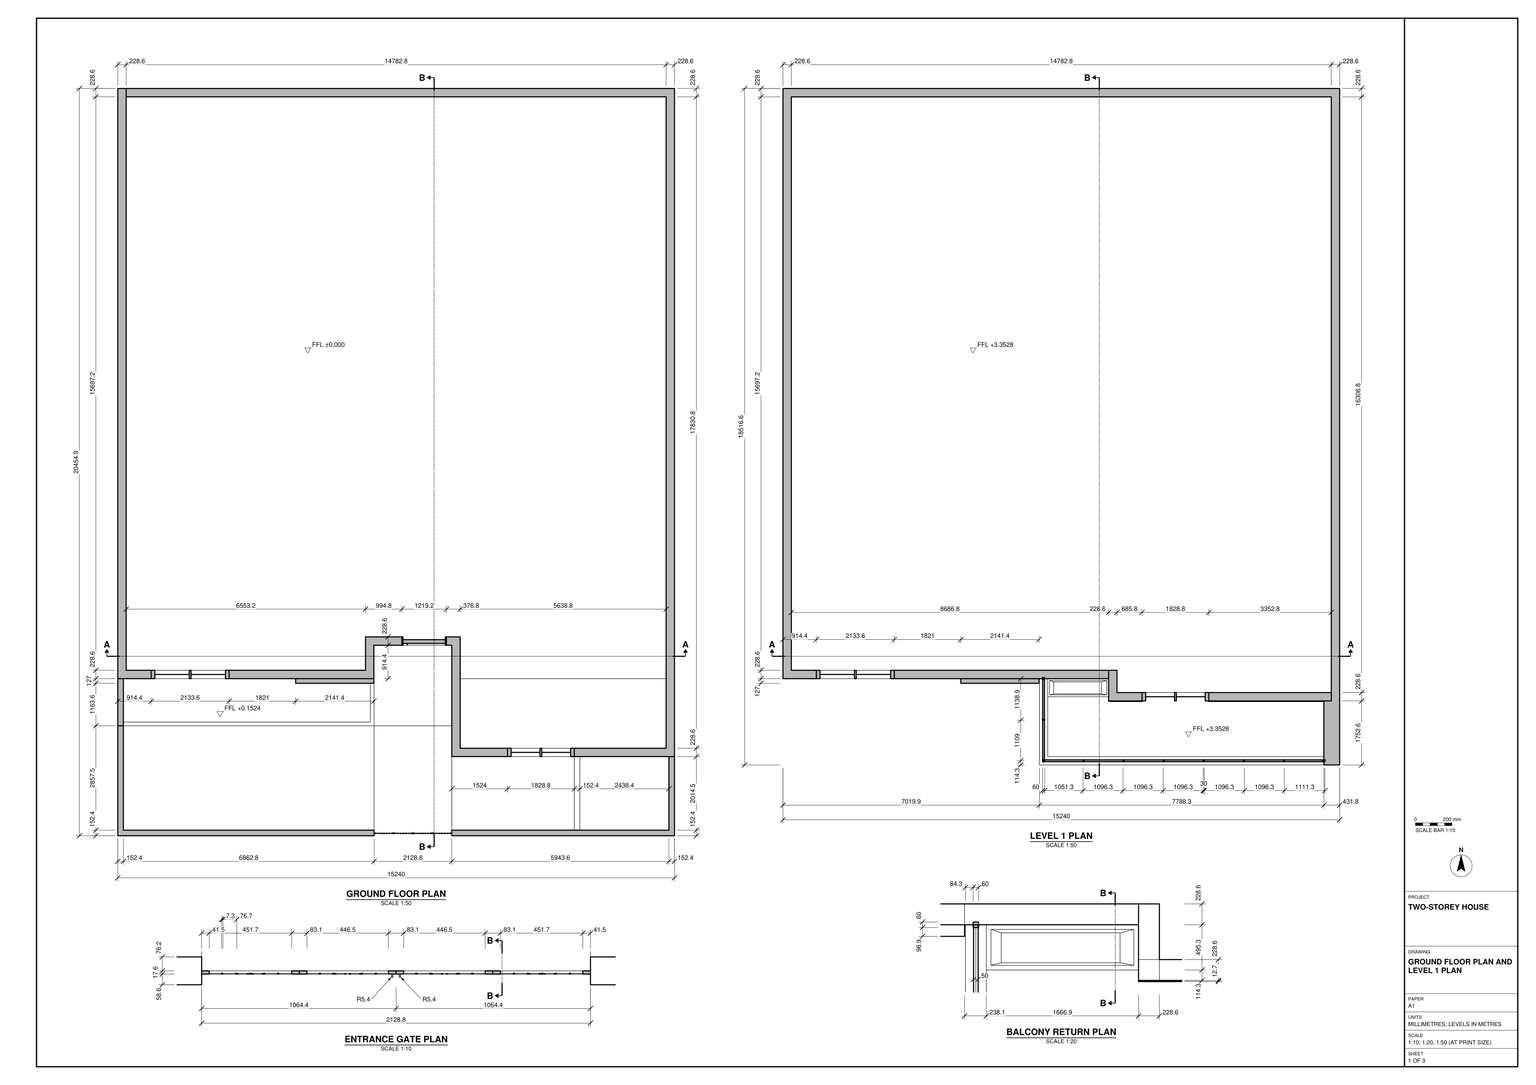
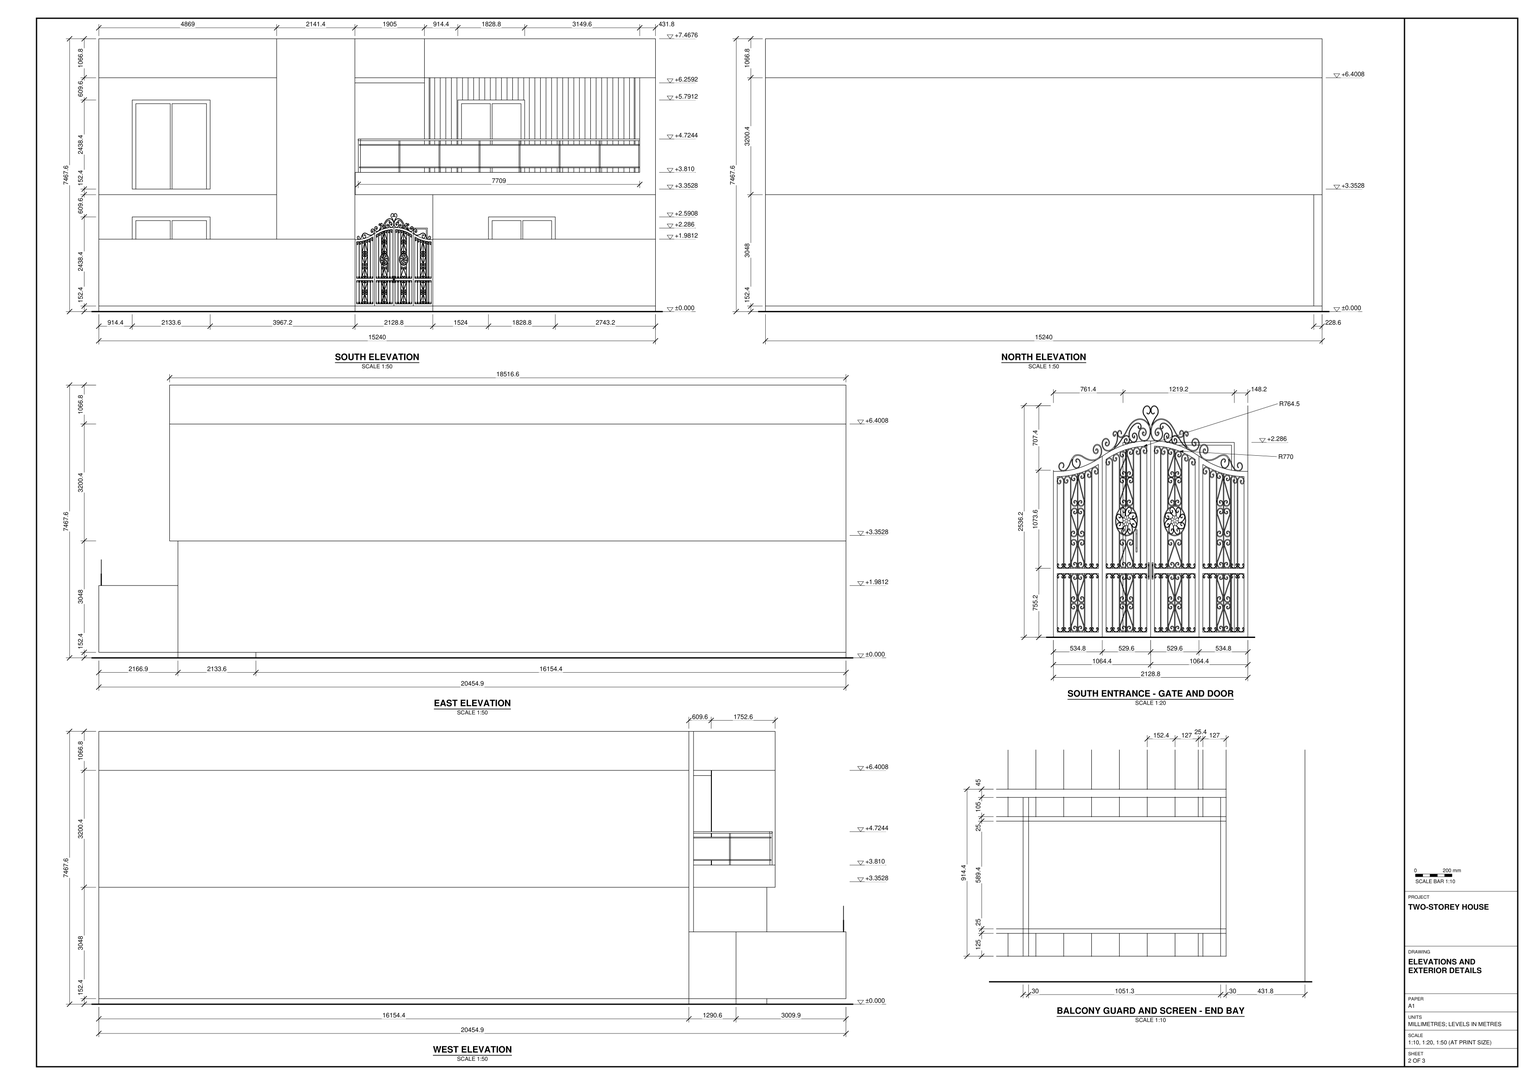
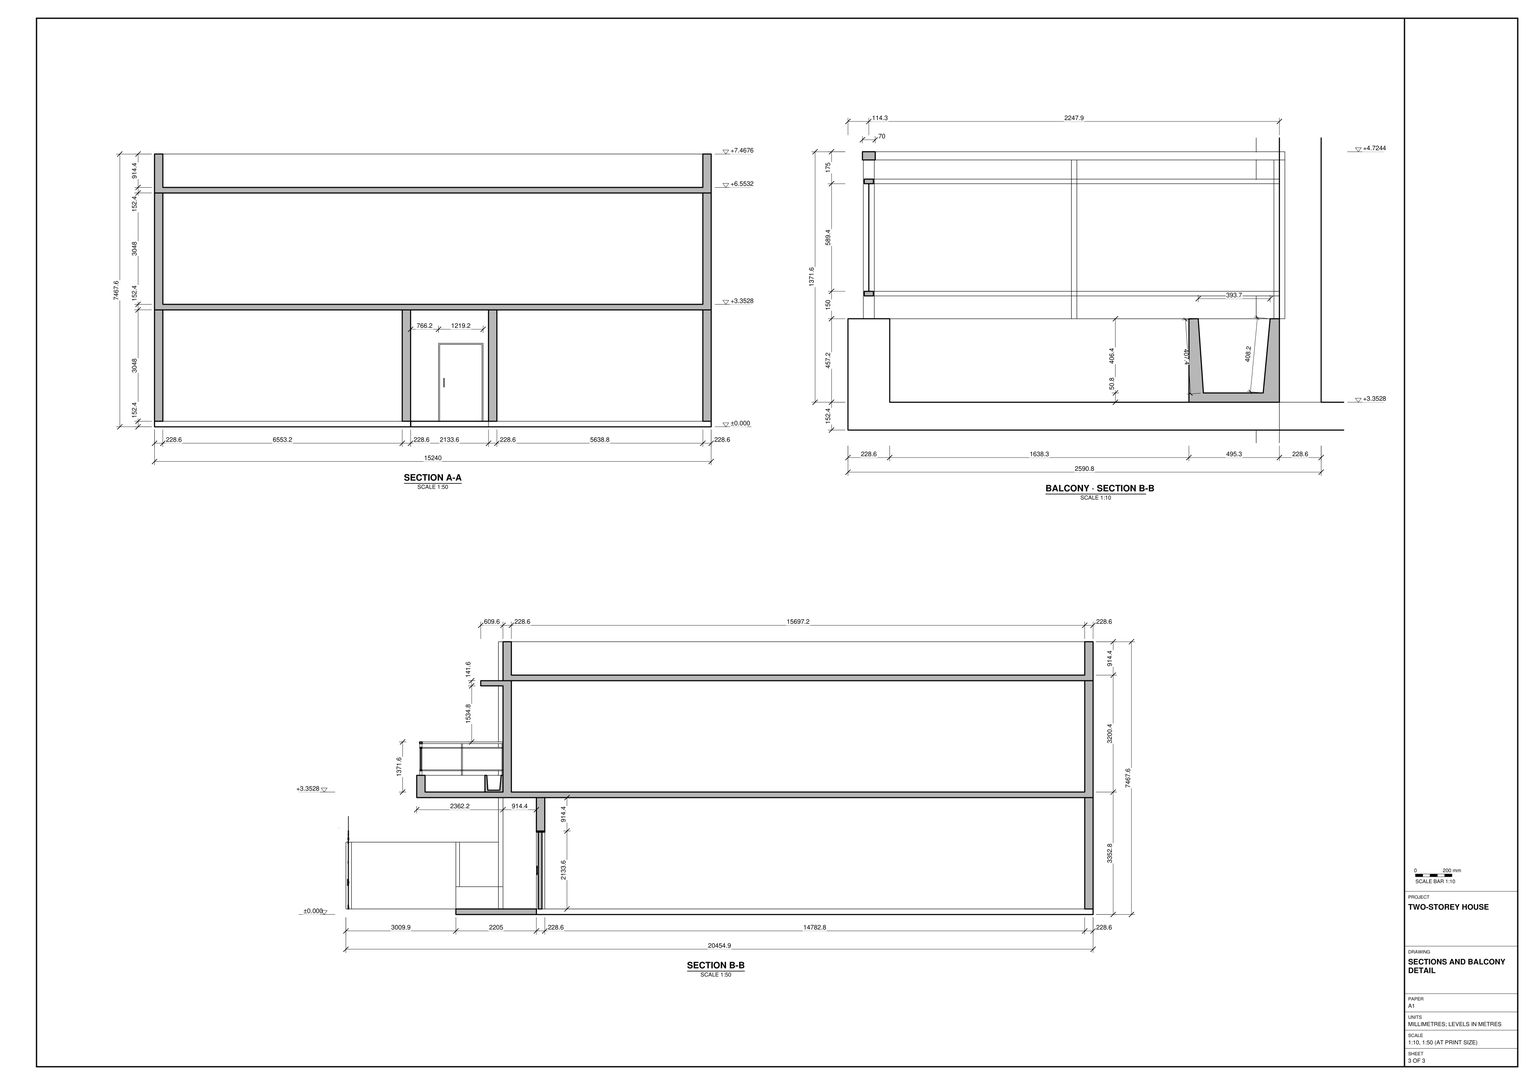
Build the house in SketchUp from task_files/diagram_01.pdf. Work in millimetres. Including the front enclosure, the model is 15240 mm wide, 20454.9 mm deep and 7467.6 mm high. Use 0 mm as the ground-floor datum and +3352.8 mm as the upper-floor level.

Follow the plans for the stepped south frontage: the entrance door sits in a recess, the eastern bay projects forward, and a double-leaf gate closes the gap between the low front walls. Model the exterior walls at their drawn thicknesses, the floor slabs, and the flat roof with its raised parapet. Keep the main floor areas open as drawn. Use the south elevation to place the framed openings on both storeys and to shape the curved crest and scrollwork of the gate.

Build the upper balcony on the eastern part of the south frontage. Use the enlarged plan and section to form the low balcony edge, the guard and its side return, and the recessed trough at the return. Include the vertical screen behind the guard. Keep shell elements and each furniture or joinery piece separate as groups or components, and use components for repeated parts. Any decor or loose items may be suitable library components. Save one SketchUp model as output_files/two_storey_house_with_a_gated_entrance_and_balcony.skp.

# SketchUp Ruby script. Lengths in millimetres.
U = 1.mm
M = Sketchup.active_model
def pt(a) = Geom::Point3d.new(a.map { |v| v * U })
def face(e, loops, mat)
  f = e.add_face(loops[0].map { |a| pt(a) })
  loops[1..].each { |l| e.add_face(l.map { |a| pt(a) }).erase! }
  f.material = f.back_material = mat if mat
  f
end
# faces: each face lists its corners as indices into pts; further lists are holes
def faces(e, pts, list, mat = nil) = list.each { |f| face(e, (f[0].is_a?(Array) ? f : [f]).map { |l| l.map { |i| pts[i] } }, mat) }
# xy, xz, yz: faces in a plane at the given z, y or x. An outline is a flat list of corners, or four numbers for a rectangle; further outlines are holes
def ring(l) = l.size == 4 ? [[l[0], l[1]], [l[2], l[1]], [l[2], l[3]], [l[0], l[3]]] : l.each_slice(2).to_a
def flat(e, list, mat, &to3) = list.each { |f| face(e, (f[0].is_a?(Array) ? f : [f]).map { |l| ring(l).map { |u, v| to3.(u, v) } }, mat) }
def xy(e, z, list, mat = nil) = flat(e, list, mat) { |x, y| [x, y, z] }
def xz(e, y, list, mat = nil) = flat(e, list, mat) { |x, z| [x, y, z] }
def yz(e, x, list, mat = nil) = flat(e, list, mat) { |y, z| [x, y, z] }
def lines(e, pts, list) = list.each { |a, b| e.add_line(pt(pts[a]), pt(pts[b])) }
# prism: a flat outline (further loops are holes) pulled along v
def prism(e, loops, v, mat = nil)
  f = face(e, loops, mat); d = Geom::Vector3d.new(v.map { |x| x * U })
  f.pushpull(f.normal.samedirection?(d) ? d.length : -d.length)
end
def box(e, o, s, mat = nil) = prism(e, [[o, [o[0] + s[0], o[1], o[2]], [o[0] + s[0], o[1] + s[1], o[2]], [o[0], o[1] + s[1], o[2]]]], [0, 0, s[2]], mat)
def at(x, y, z, deg = 0) = Geom::Transformation.translation(pt([x, y, z])) * Geom::Transformation.rotation(ORIGIN, Z_AXIS, deg.degrees)
def axes(o, x, y, z) = Geom::Transformation.new([*x, 0, *y, 0, *z, 0, *pt(o).to_a, 1])
def part(name) = M.definitions.add(name)
# library, detail: a bought-in or finely detailed component or shape, given as its bounding box
def library(name, o, s) = part(name).tap { |d| box(d.entities, o, s) }
def detail(e, o, s) = box(e.add_group.entities, o, s)
def put(e, d, t, mat = nil) = e.add_instance(d, t).tap { |i| i.material = mat if mat }
def group(e, t, mat = nil) = e.add_group.tap { |g| g.transformation = t; g.material = mat if mat }.entities
root = M.entities
M.materials.add("CLC2-HANDLES-BT - LANSA").color = [177, 177, 177]
M.materials.add("Calacatta Gold (48O4VB)").color = [235, 228, 225]
M.materials.add("[Color B01]").color = [99, 67, 51]
M.materials.add("[Color C01]").color = [255, 229, 204]
M.materials.add("[Color C07]").color = [153, 76, 0]
M.materials.add("[Color E01]").color = [73, 76, 82]
M.materials.add("[Color M09]").color = [0, 0, 0]
M.materials.add("[Grass Light Green]").color = [138, 158, 69]
M.materials.add("[Translucent Glass Gray]").color = [128, 128, 128]
M.materials["[Translucent Glass Gray]"].alpha = 0.5
M.materials.add("[Wood Floor]").color = [155, 105, 61]
M.materials.add("[Wood Veneer 01]").color = [120, 70, 37]
c1 = library("Ornamental gate leaf",[0,0,0],[4100,1077.8,7119.6])
c2 = part("cong")
put(c2.entities,c1,axes([6217.3,5957.9,0],[-1,0,0],[0,1,0],[0,0,1]))
put(c2.entities,c1,at(6217.3,5957.9,0))
c3 = part("3-POIGNEE CLC2")
yz(c3.entities,-122.5,[[0,28,-1.68,28.22,-3.25,28.87,-4.6,29.9,-5.63,31.25,-6.28,32.82,-6.5,34.5,-6.28,36.18,-5.63,37.75,-4.6,39.1,-3.25,40.13,-1.68,40.78,0,41,1.68,40.78,3.25,40.13,4.6,39.1,5.63,37.75,6.28,36.18,6.5,34.5,6.28,32.82,5.63,31.25,4.6,29.9,3.25,28.87,1.68,28.22]],"CLC2-HANDLES-BT - LANSA")
yz(c3.entities,122.5,[[0,28,1.68,28.22,3.25,28.87,4.6,29.9,5.63,31.25,6.28,32.82,6.5,34.5,6.28,36.18,5.63,37.75,4.6,39.1,3.25,40.13,1.68,40.78,0,41,-1.68,40.78,-3.25,40.13,-4.6,39.1,-5.63,37.75,-6.28,36.18,-6.5,34.5,-6.28,32.82,-5.63,31.25,-4.6,29.9,-3.25,28.87,-1.68,28.22]],"CLC2-HANDLES-BT - LANSA")
p = [[-77.37,-4.5,29.84],[-78.54,-4.38,29.75],[-78.54,-4.38,0],[-77.63,-4.47,0],[-77.37,-4.5,0],[-76.21,-4.31,0],
  [-76.21,-4.31,29.7],[77.63,-4.5,29.84],[76.46,-4.38,29.75],[76.46,-4.38,0],[77.37,-4.47,0],[77.63,-4.5,0],
  [78.79,-4.31,0],[78.79,-4.31,29.7],[-79.64,-3.96,29.43],[-79.64,-3.96,0],[75.36,-3.96,29.43],[75.36,-3.96,0],
  [-75.14,-3.83,0],[-75.14,-3.83,29.33],[79.86,-3.83,0],[79.86,-3.83,29.33],[-80.59,-3.27,28.9],[-80.59,-3.26,28.87],
  [-80.59,-3.27,0],[74.41,-3.27,28.9],[74.41,-3.27,0],[-74.23,-3.09,0],[-74.23,-3.09,28.81],[-74.41,-3.24,28.87],
  [80.77,-3.09,0],[80.77,-3.09,28.81],[80.59,-3.24,28.87],[-80.61,-3.25,28.88],[-81.33,-2.36,28.51],[-81.33,-2.36,0],
  [74.39,-3.24,28.88],[73.67,-2.36,28.51],[73.67,-2.36,0],[-73.54,-2.14,0],[-73.54,-2.14,28.41],[81.46,-2.14,0],
  [81.46,-2.14,28.41],[-81.64,-1.67,28.22],[-81.81,-1.29,28.17],[-81.81,-1.29,0],[73.36,-1.67,28.22],[73.19,-1.29,28.17],
  [73.19,-1.29,0],[-73.12,-1.04,0],[-73.12,-1.04,28.14],[-73.36,-1.67,28.22],[81.88,-1.04,0],[81.88,-1.04,28.14],
  [81.64,-1.67,28.22],[-82,-0.13,28.02],[-82,-0.13,0],[73,-0.13,28.02],[73,-0.13,0],[-73,0.13,0],
  [-73,0.13,28.02],[-73.01,0.01,28],[82,0.13,0],[82,0.13,28.02],[81.99,0.01,28],[-81.98,0.01,28],
  [-81.88,1.04,28.13],[-81.88,1.04,0],[73.02,0.01,28],[73.12,1.04,28.13],[73.12,1.04,0],[-73.19,1.29,0],
  [-73.19,1.29,28.17],[81.81,1.29,0],[81.81,1.29,28.17],[-81.63,1.7,28.22],[-81.46,2.14,28.4],[-81.46,2.14,0],
  [73.37,1.7,28.22],[73.54,2.14,28.4],[73.54,2.14,0],[-73.67,2.36,0],[-73.67,2.36,28.5],[-73.37,1.7,28.22],
  [81.33,2.36,0],[81.33,2.36,28.5],[81.63,1.7,28.22],[-80.77,3.09,28.8],[-80.77,3.09,0],[74.23,3.09,28.8],
  [74.23,3.09,0],[-74.41,3.27,0],[-74.41,3.27,28.88],[-74.39,3.25,28.87],[80.59,3.27,0],[80.59,3.27,28.88],
  [80.61,3.25,28.87],[-80.56,3.26,28.87],[-79.86,3.83,29.31],[-79.86,3.83,0],[74.44,3.26,28.87],[75.14,3.83,29.31],
  [75.14,3.83,0],[-75.36,3.96,0],[-75.36,3.96,29.41],[79.64,3.96,0],[79.64,3.96,29.41],[-78.79,4.31,29.67],
  [-78.79,4.31,0],[76.21,4.31,29.67],[76.21,4.31,0],[-76.46,4.38,0],[-76.46,4.38,29.73],[78.54,4.38,0],
  [78.54,4.38,29.73],[-77.63,4.5,29.82],[-77.63,4.5,0],[77.37,4.5,29.82],[77.37,4.5,0],[-122.5,0,28],
  [-122.5,-1.68,28.22],[122.5,-1.68,28.22],[122.5,0,28],[-122.5,1.68,28.22],[122.5,1.68,28.22],[122.5,-3.25,28.87],
  [-122.5,-3.25,28.87],[89.32,3.25,28.87],[122.5,3.25,28.87],[-122.5,3.25,28.87],[122.5,-4.6,29.9],[-122.5,-4.6,29.9],
  [122.5,4.6,29.9],[-122.5,4.6,29.9],[-122.5,-5.63,31.25],[122.5,-5.63,31.25],[-122.5,5.63,31.25],[122.5,5.63,31.25],
  [-122.5,-6.28,32.82],[122.5,-6.28,32.82],[-122.5,6.28,32.82],[122.5,6.28,32.82],[-122.5,-6.5,34.5],[122.5,-6.5,34.5],
  [-122.5,6.5,34.5],[122.5,6.5,34.5],[-122.5,-6.28,36.18],[122.5,-6.28,36.18],[-122.5,6.28,36.18],[122.5,6.28,36.18],
  [-122.5,-5.63,37.75],[122.5,-5.63,37.75],[-122.5,5.63,37.75],[122.5,5.63,37.75],[-122.5,-4.6,39.1],[122.5,-4.6,39.1],
  [-122.5,4.6,39.1],[122.5,4.6,39.1],[-122.5,-3.25,40.13],[122.5,-3.25,40.13],[-122.5,3.25,40.13],[122.5,3.25,40.13],
  [-122.5,-1.68,40.78],[122.5,-1.68,40.78],[-122.5,1.68,40.78],[122.5,1.68,40.78],[-122.5,0,41],[122.5,0,41]]
faces(c3.entities,p,[[0,1,2,3,4],[5,6,0,4],[7,8,9,10,11],[12,13,7,11],[2,1,14,15],[9,8,16,17],[18,19,6,5],[20,21,13,12],
  [15,14,22,23,24],[17,16,25,26],[27,28,29,19,18],[30,31,32,21,20],[24,23,22,33,34,35],[26,25,36,37,38],[39,40,28,27],[41,42,31,30],
  [35,34,43,44,45],[38,37,46,47,48],[49,50,51,40,39],[52,53,54,42,41],[45,44,55,56],[48,47,57,58],[59,60,61,50,49],[62,63,64,53,52],
  [56,55,65,66,67],[58,57,68,69,70],[71,72,60,59],[73,74,63,62],[67,66,75,76,77],[70,69,78,79,80],[81,82,83,72,71],[84,85,86,74,73],
  [77,76,87,88],[80,79,89,90],[91,92,93,82,81],[94,95,96,85,84],[88,87,97,98,99],[90,89,100,101,102],[103,104,92,91],[105,106,95,94],
  [99,98,107,108],[102,101,109,110],[111,112,104,103],[113,114,106,105],[108,107,115,116],[110,109,117,118],[116,115,112,111],[118,117,114,113],
  [119,65,55,44,43,120],[65,61,50,51,43,44,55],[61,68,57,47,46,51,50],[68,64,53,54,46,47,57],[121,54,53,64,122],[123,75,66,65,119],[75,83,72,60,61,65,66],[83,78,69,68,61,60,72],
  [64,68,69,78,86,74,63],[122,64,63,74,86,124],[120,43,51,46,54,121,125,32,36,29,33,126],[127,128,124,86,78,83,75,123,129,97,92,100,95],[126,33,29,36,32,125,130,131],[132,128,127,95,100,92,97,129,133],[134,131,130,135],[133,136,137,132],
  [138,134,135,139],[136,140,141,137],[142,138,139,143],[140,144,145,141],[146,142,143,147],[144,148,149,145],[150,146,147,151],[148,152,153,149],
  [154,150,151,155],[152,156,157,153],[158,154,155,159],[156,160,161,157],[162,158,159,163],[160,164,165,161],[166,162,163,167],[164,166,167,165]],"CLC2-HANDLES-BT - LANSA")
c4 = part("Group22\#2")
xy(c4.entities,0,[[0,0,789.8,2338.4]],"[Translucent Glass Gray]")
c5 = part("Group20\#1")
xy(c5.entities,0,[[0,0,0,2438.4,1828.8,2438.4,1828.8,0,1728.8,0,1728.8,2338.4,939,2338.4,939,0,889.8,0,889.8,2338.4,100,2338.4,100,0]])
xy(c5.entities,228.6,[[0,0,100,0,100,2338.4,889.8,2338.4,889.8,0,939,0,939,2338.4,1728.8,2338.4,1728.8,0,1828.8,0,1828.8,2438.4,0,2438.4]],"[Wood Veneer 01]")
xz(c5.entities,0,[[0,0,100,228.6],[889.8,0,939,228.6],[1728.8,0,1828.8,228.6]])
xz(c5.entities,2338.4,[[100,0,889.8,228.6],[939,0,1728.8,228.6]])
xz(c5.entities,2438.4,[[0,0,1828.8,228.6]])
yz(c5.entities,0,[[0,0,2438.4,228.6]])
yz(c5.entities,100,[[0,0,2338.4,228.6]])
yz(c5.entities,889.8,[[0,0,2338.4,228.6]])
yz(c5.entities,939,[[0,0,2338.4,228.6]])
yz(c5.entities,1728.8,[[0,0,2338.4,228.6]])
yz(c5.entities,1828.8,[[0,0,2438.4,228.6]])
p = [[889.8,0,0],[100,0,0],[1728.8,0,0],[939,0,0],[2,2,0],[2,2,228.6]]
lines(c5.entities,p,[[0,1],[2,3],[4,5]])
put(c5.entities,c4,at(100,0,114.3))
put(c5.entities,c4,at(939,0,114.3))
c6 = part("Group24\#2")
xy(c6.entities,0,[[0,0,942.2,2338.4]],"[Translucent Glass Gray]")
c7 = part("Group22\#1")
prism(c7.entities,[[[2133.6,2438.4,0],[2133.6,0,0],[2033.6,0,0],[2033.6,2338.4,0],[1091.4,2338.4,0],[1091.4,0,0],[1042.2,0,0],[1042.2,2338.4,0],[100,2338.4,0],[100,0,0],[0,0,0],[0,2438.4,0]]],[0,0,228.6],"[Wood Veneer 01]")
p = [[1042.2,0,0],[100,0,0],[2033.6,0,0],[1091.4,0,0],[2,2,0],[2,2,228.6]]
lines(c7.entities,p,[[0,1],[2,3],[4,5]])
put(c7.entities,c6,at(100,0,114.3))
put(c7.entities,c6,at(1091.4,0,114.3))
c8 = part("Group27\#1")
box(c8.entities,[0,-5664.2,0],[3048,152.4,12.7])
c9 = part("Group28\#1")
prism(c9.entities,[[[3048,76.2,0],[0,76.2,0],[0,228.6,0],[2906.4,228.6,0],[3048,228.6,0]]],[0,0,12.7])
c10 = part("Group29\#1")
box(c10.entities,[0,-2794,0],[3048,152.4,12.7])
c11 = part("Group30\#1")
box(c11.entities,[0,-2946.4,0],[3048,152.4,12.7])
c12 = part("Group31\#1")
xy(c12.entities,0,[[0,-2641.6,0,-2514.6,2438.4,-2514.6,2438.4,-2489.2,3048,-2489.2,3048,-2641.6]])
xy(c12.entities,12.7,[[0,-2641.6,3048,-2641.6,3048,-2489.2,2438.4,-2489.2,2438.4,-2514.6,0,-2514.6]])
xz(c12.entities,-2641.6,[[0,0,3048,12.7]])
xz(c12.entities,-2489.2,[[2438.4,0,3048,12.7]])
yz(c12.entities,3048,[[-2641.6,0,-2489.2,12.7]])
c13 = part("Group32\#1")
box(c13.entities,[0,-3098.8,0],[3048,152.4,12.7])
c14 = part("Group33\#1")
box(c14.entities,[2438.4,-2489.2,0],[609.6,152.4,12.7])
c15 = part("Group34\#1")
box(c15.entities,[0,-3251.2,0],[3048,152.4,12.7])
c16 = part("Group35\#1")
box(c16.entities,[2438.4,-2336.8,0],[609.6,152.4,12.7])
c17 = part("Group36\#1")
box(c17.entities,[0,-3403.6,0],[3048,152.4,12.7])
c18 = part("Group37\#1")
box(c18.entities,[2438.4,-2184.4,0],[609.6,152.4,12.7])
c19 = part("Group38\#1")
box(c19.entities,[0,-3556,0],[3048,152.4,12.7])
c20 = part("Group39\#1")
box(c20.entities,[2438.4,-2032,0],[609.6,152.4,12.7])
c21 = part("Group40\#1")
box(c21.entities,[0,-3708.4,0],[3048,152.4,12.7])
c22 = part("Group41\#1")
box(c22.entities,[2438.4,-1879.6,0],[609.6,152.4,12.7])
c23 = part("Group42\#1")
box(c23.entities,[0,-3860.8,0],[3048,152.4,12.7])
c24 = part("Group43\#1")
box(c24.entities,[2438.4,-1727.2,0],[609.6,152.4,12.7])
c25 = part("Group44\#1")
box(c25.entities,[0,-4013.2,0],[3048,152.4,12.7])
c26 = part("Group45\#1")
box(c26.entities,[2438.4,-1574.8,0],[609.6,152.4,12.7])
c27 = part("Group46\#1")
box(c27.entities,[0,-4165.6,0],[3048,152.4,12.7])
c28 = part("Group47\#1")
box(c28.entities,[2438.4,-1422.4,0],[609.6,152.4,12.7])
c29 = part("Group48\#1")
box(c29.entities,[0,-4318,0],[3048,152.4,12.7])
c30 = part("Group49\#1")
box(c30.entities,[2438.4,-1270,0],[609.6,152.4,12.7])
c31 = part("Group50\#1")
box(c31.entities,[0,-4470.4,0],[3048,152.4,12.7])
c32 = part("Group51\#1")
box(c32.entities,[2438.4,-1117.6,0],[609.6,152.4,12.7])
c33 = part("Group52\#1")
box(c33.entities,[0,-4622.8,0],[3048,152.4,12.7])
c34 = part("Group53\#1")
box(c34.entities,[2438.4,-965.2,0],[609.6,152.4,12.7])
c35 = part("Group54\#1")
box(c35.entities,[0,-4775.2,0],[3048,152.4,12.7])
c36 = part("Group55\#1")
xy(c36.entities,0,[[2438.4,-812.8,2438.4,-685.8,0,-685.8,0,-660.4,3048,-660.4,3048,-812.8]])
xy(c36.entities,12.7,[[2438.4,-812.8,3048,-812.8,3048,-660.4,0,-660.4,0,-685.8,2438.4,-685.8]])
xz(c36.entities,-812.8,[[2438.4,0,3048,12.7]])
xz(c36.entities,-660.4,[[0,0,3048,12.7]])
yz(c36.entities,3048,[[-812.8,0,-660.4,12.7]])
c37 = part("Group56\#1")
box(c37.entities,[0,-4927.6,0],[3048,152.4,12.7])
c38 = part("Group57\#1")
box(c38.entities,[0,-660.4,0],[3048,152.4,12.7])
c39 = part("Group58\#1")
box(c39.entities,[0,-5080,0],[3048,152.4,12.7])
c40 = part("Group59\#1")
box(c40.entities,[0,-508,0],[3048,152.4,12.7])
c41 = part("Group60\#1")
box(c41.entities,[0,-5232.4,0],[3048,152.4,12.7])
c42 = part("Group61\#1")
box(c42.entities,[0,-355.6,0],[3048,152.4,12.7])
c43 = part("Group62\#1")
box(c43.entities,[0,-5384.8,0],[3048,152.4,12.7])
c44 = part("Group63\#1")
box(c44.entities,[0,-203.2,0],[3048,152.4,12.7])
c45 = part("Group64\#1")
box(c45.entities,[0,-5537.2,0],[3048,152.4,12.7])
c46 = part("Group65\#1")
xy(c46.entities,0,[[0,-50.8,3048,101.6]])
xy(c46.entities,12.7,[[0,-50.8,3048,101.6]])
xz(c46.entities,-50.8,[[0,0,3048,12.7]])
xz(c46.entities,101.6,[[0,0,3048,12.7]])
yz(c46.entities,0,[[-50.8,0,101.6,12.7]])
yz(c46.entities,3048,[[-50.8,0,101.6,12.7]])
c47 = part("Group25\#1")
put(c47.entities,c8,at(0,0,0))
put(c47.entities,c9,at(0,0,0))
put(c47.entities,c10,at(0,0,0))
put(c47.entities,c11,at(0,0,0))
put(c47.entities,c12,at(0,0,0))
put(c47.entities,c13,at(0,0,0))
put(c47.entities,c14,at(0,0,0))
put(c47.entities,c15,at(0,0,0))
put(c47.entities,c16,at(0,0,0))
put(c47.entities,c17,at(0,0,0))
put(c47.entities,c18,at(0,0,0))
put(c47.entities,c19,at(0,0,0))
put(c47.entities,c20,at(0,0,0))
put(c47.entities,c21,at(0,0,0))
put(c47.entities,c22,at(0,0,0))
put(c47.entities,c23,at(0,0,0))
put(c47.entities,c24,at(0,0,0))
put(c47.entities,c25,at(0,0,0))
put(c47.entities,c26,at(0,0,0))
put(c47.entities,c27,at(0,0,0))
put(c47.entities,c28,at(0,0,0))
put(c47.entities,c29,at(0,0,0))
put(c47.entities,c30,at(0,0,0))
put(c47.entities,c31,at(0,0,0))
put(c47.entities,c32,at(0,0,0))
put(c47.entities,c33,at(0,0,0))
put(c47.entities,c34,at(0,0,0))
put(c47.entities,c35,at(0,0,0))
put(c47.entities,c36,at(0,0,0))
put(c47.entities,c37,at(0,0,0))
put(c47.entities,c38,at(0,0,0))
put(c47.entities,c39,at(0,0,0))
put(c47.entities,c40,at(0,0,0))
put(c47.entities,c41,at(0,0,0))
put(c47.entities,c42,at(0,0,0))
put(c47.entities,c43,at(0,0,0))
put(c47.entities,c44,at(0,0,0))
put(c47.entities,c45,at(0,0,0))
put(c47.entities,c46,at(0,0,0))
c48 = part("Group95\#1")
box(c48.entities,[7104.2,3787.9,3810],[60,60,869.4])
c49 = part("Group96\#1")
box(c49.entities,[7104.2,1540,3810],[60,60,869.4])
c50 = part("Group97\#1")
box(c50.entities,[7104.2,2679,3810],[60,30,869.4])
c51 = part("Group98\#1")
box(c51.entities,[7099.2,1540,4679.4],[70,2307.9,45])
c52 = part("Group99\#1")
box(c52.entities,[7109.2,1570,4549.4],[50,2247.9,25])
c53 = part("Group100\#1")
box(c53.entities,[7109.2,1570,3935],[50,2247.9,25])
c54 = part("Group101\#1")
yz(c54.entities,7134.2,[[1570,3960,3817.9,4549.4]],"[Translucent Glass Gray]")
c55 = part("Group103\#2")
box(c55.entities,[14778.2,1540,3810],[60,60,869.4])
c56 = part("Group104\#1")
box(c56.entities,[8215.5,1540,3810],[30,60,869.4])
box(c56.entities,[9311.8,1540,3810],[30,60,869.4])
box(c56.entities,[10408.1,1540,3810],[30,60,869.4])
box(c56.entities,[11504.4,1540,3810],[30,60,869.4])
box(c56.entities,[12600.6,1540,3810],[30,60,869.4])
box(c56.entities,[13696.9,1540,3810],[30,60,869.4])
c57 = part("Group105\#1")
box(c57.entities,[7104.2,1535,4679.4],[7734,70,45])
c58 = part("Group106\#1")
box(c58.entities,[7134.2,1545,4549.4],[7674,50,25])
c59 = part("Group107\#1")
box(c59.entities,[7134.2,1545,3935],[7674,50,25])
c60 = part("Group108\#1")
xz(c60.entities,1570,[[7134.2,3960,14808.2,4549.4]],"[Translucent Glass Gray]")
c61 = part("Component\#1")
xy(c61.entities,0,[[7019.9,-228.6,7019.9,2133.6,0,2133.6,0,18288,15240,18288,15240,-228.6]],"[Color C01]")
xy(c61.entities,152.4,[[7248.5,0,14808.2,0,14808.2,1524,11658.6,1524,11658.6,1752.6,9829.8,1752.6,9829.8,1524,8915.4,1524,8915.4,2133.6,7248.5,2133.6],[9144,1524,9829.8,1752.6],[11658.6,1524,15011.4,1752.6],[9144,1752.6,15011.4,1752.6,15011.4,18059.4,228.6,18059.4,228.6,2362.2,9144,2362.2],[8915.4,1752.6,9144,2362.2],
  [914.4,2133.6,3048,2362.2]],"[Color C01]")
xy(c61.entities,609.6,[[7019.9,-228.6,14808.2,-228.6,14808.2,-114.3,7134.2,-114.3,7134.2,2133.6,7019.9,2133.6],[7134.2,-114.3,14808.2,-114.3,14808.2,0,7248.5,0,7248.5,2133.6,7134.2,2133.6]],"[Color C01]")
xy(c61.entities,2590.8,[[9829.8,1524,11658.6,1752.6],[914.4,2133.6,3048,2362.2]],"[Color C01]")
xy(c61.entities,3058.8,[[7010.4,1524,8915.4,2133.6]],"[Color C01]")
xy(c61.entities,3200.4,[[14808.2,-228.6,15240,-228.6,15240,18288,0,18288,0,2133.6,7010.4,2133.6,7010.4,1524,8915.4,1524,8915.4,2362.2,228.6,2362.2,228.6,18059.4,15011.4,18059.4,15011.4,1524,14808.2,1524],[8915.4,1524,15011.4,1524,15011.4,1752.6,9144,1752.6,9144,2362.2,8915.4,2362.2]],"[Color C01]")
xz(c61.entities,-228.6,[[7019.9,0,15240,0,15240,3200.4,14808.2,3200.4,14808.2,609.6,7019.9,609.6]],"[Color C01]")
xz(c61.entities,0,[[7248.5,152.4,14808.2,609.6],[14808.2,152.4,15011.4,609.6]],"[Color C01]")
xz(c61.entities,1524,[[8915.4,152.4,9829.8,152.4,9829.8,2590.8,11658.6,2590.8,11658.6,152.4,14808.2,152.4,14808.2,3200.4,8915.4,3200.4],[14808.2,152.4,15011.4,3200.4],[7010.4,3058.8,8915.4,3200.4]],"[Color C01]")
xz(c61.entities,1752.6,[[9144,152.4,9144,3200.4,15011.4,3200.4,15011.4,152.4,11658.6,152.4,11658.6,2590.8,9829.8,2590.8,9829.8,152.4]],"[Color C01]")
xz(c61.entities,2133.6,[[[0,0,7019.9,0,7019.9,609.6,7248.5,609.6,7248.5,152.4,8915.4,152.4,8915.4,3058.8,7010.4,3058.8,7010.4,3200.4,0,3200.4],[914.4,152.4,3048,2590.8]]],"[Color C01]")
xz(c61.entities,2362.2,[[228.6,152.4,228.6,3200.4,8915.4,3200.4,8915.4,152.4,3048,152.4,3048,2590.8,914.4,2590.8,914.4,152.4],[8915.4,152.4,9144,3200.4]],"[Color C01]")
xz(c61.entities,18059.4,[[228.6,152.4,15011.4,3200.4]],"[Color C01]")
xz(c61.entities,18288,[[0,0,15240,3200.4]],"[Color C01]")
yz(c61.entities,0,[[2133.6,0,18288,3200.4]],"[Color C01]")
yz(c61.entities,228.6,[[2362.2,152.4,18059.4,3200.4]],"[Color C01]")
yz(c61.entities,914.4,[[2133.6,152.4,2362.2,2590.8]],"[Color C01]")
yz(c61.entities,3048,[[2133.6,152.4,2362.2,2590.8]],"[Color C01]")
yz(c61.entities,7010.4,[[1524,3058.8,2133.6,3200.4]],"[Color C01]")
yz(c61.entities,7019.9,[[-228.6,0,2133.6,609.6]],"[Color C01]")
yz(c61.entities,7248.5,[[0,152.4,2133.6,609.6]],"[Color C01]")
yz(c61.entities,8915.4,[[1524,152.4,2133.6,3058.8],[2133.6,152.4,2133.6,3058.8,1524,3058.8,1524,3200.4,2362.2,3200.4,2362.2,152.4]],"[Color C01]")
yz(c61.entities,9144,[[1752.6,152.4,2362.2,3200.4]],"[Color C01]")
yz(c61.entities,9829.8,[[1524,152.4,1752.6,2590.8]],"[Color C01]")
yz(c61.entities,11658.6,[[1524,152.4,1752.6,2590.8]],"[Color C01]")
yz(c61.entities,14808.2,[[0,152.4,0,609.6,-228.6,609.6,-228.6,3200.4,1524,3200.4,1524,152.4]],"[Color C01]")
yz(c61.entities,15011.4,[[1524,152.4,1752.6,3200.4],[1752.6,152.4,18059.4,3200.4]],"[Color C01]")
yz(c61.entities,15240,[[-228.6,0,18288,3200.4]],"[Color C01]")
p = [[15011.4,0,609.6],[15011.4,-228.6,609.6],[15011.4,0,152.4],[15011.4,-228.6,152.4]]
lines(c61.entities,p,[[0,1],[2,3]])
put(c61.entities,c5,axes([9829.8,1752.6,152.4],[1,0,0],[0,0,1],[0,-1,0]))
put(c61.entities,c7,axes([914.4,2362.2,152.4],[1,0,0],[0,0,1],[0,-1,0]))
put(c61.entities,c47,axes([9144,1524,152.4],[0,0,1],[-1,0,0],[0,-1,0]),"[Wood Floor]")
put(c61.entities,c48,at(0,-1684.3,-3200.4),"[Color M09]")
put(c61.entities,c49,at(0,-1684.3,-3200.4),"[Color M09]")
put(c61.entities,c50,at(0,-1684.3,-3200.4),"[Color M09]")
put(c61.entities,c51,at(0,-1684.3,-3200.4),"[Color M09]")
put(c61.entities,c52,at(0,-1684.3,-3200.4),"[Color M09]")
put(c61.entities,c53,at(0,-1684.3,-3200.4),"[Color M09]")
put(c61.entities,c54,at(0,-1684.3,-3200.4))
put(c61.entities,c55,at(0,-1684.3,-3200.4))
put(c61.entities,c56,at(0,-1684.3,-3200.4),"[Color M09]")
put(c61.entities,c57,at(0,-1684.3,-3200.4),"[Color M09]")
put(c61.entities,c58,at(0,-1684.3,-3200.4),"[Color M09]")
put(c61.entities,c59,at(0,-1684.3,-3200.4),"[Color M09]")
put(c61.entities,c60,at(0,-1684.3,-3200.4))
c62 = part("Group10\#1")
prism(c62.entities,[[[609.6,1066.8,0],[609.6,-1066.8,0],[579.4,-1066.8,0],[579.4,1036.6,0],[-579.4,1036.6,0],[-579.4,-1066.8,0],[-609.6,-1066.8,0],[-609.6,1066.8,0]]],[0,0,228.6])
c63 = part("Group17\#2")
xy(c63.entities,0,[[0,0,942.2,2338.4]],"[Translucent Glass Gray]")
c64 = part("Group15\#1")
prism(c64.entities,[[[2133.6,2438.4,0],[2133.6,0,0],[2033.6,0,0],[2033.6,2338.4,0],[1091.4,2338.4,0],[1091.4,0,0],[1042.2,0,0],[1042.2,2338.4,0],[100,2338.4,0],[100,0,0],[0,0,0],[0,2438.4,0]]],[0,0,228.6],"[Wood Veneer 01]")
p = [[2033.6,0,0],[1091.4,0,0],[1042.2,0,0],[100,0,0],[2,2,0],[2,2,228.6]]
lines(c64.entities,p,[[0,1],[2,3],[4,5]])
put(c64.entities,c63,at(100,0,114.3))
put(c64.entities,c63,at(1091.4,0,114.3))
c65 = part("Group19\#2")
xy(c65.entities,0,[[0,0,789.8,2338.4]],"[Translucent Glass Gray]")
c66 = part("Group17\#1")
prism(c66.entities,[[[1828.8,2438.4,0],[1828.8,0,0],[1728.8,0,0],[1728.8,2338.4,0],[939,2338.4,0],[939,0,0],[889.8,0,0],[889.8,2338.4,0],[100,2338.4,0],[100,0,0],[0,0,0],[0,2438.4,0]]],[0,0,228.6],"[Wood Veneer 01]")
p = [[889.8,0,0],[100,0,0],[1728.8,0,0],[939,0,0],[2,2,0],[2,2,228.6]]
lines(c66.entities,p,[[0,1],[2,3],[4,5]])
put(c66.entities,c65,at(100,0,114.3))
put(c66.entities,c65,at(939,0,114.3))
c67 = part("Group14\#1")
xy(c67.entities,152.4,[[12496.8,1684.3,12496.8,1912.9,15011.4,1912.9,15011.4,19743.7,228.6,19743.7,228.6,19972.3,15240,19972.3,15240,1684.3],[9144,1684.3,9144,4732.3,8995.8,4732.3,8995.8,4960.9,9372.6,4960.9,9372.6,1912.9,10668,1912.9,10668,1684.3],[0,3817.9,0,19972.3,228.6,19972.3,228.6,4046.5,914.4,4046.5,914.4,3817.9],[3048,3817.9,3048,4046.5,6781.8,4046.5,6781.8,4960.9,7776.6,4960.9,7776.6,4732.3,7010.4,4732.3,7010.4,3817.9]])
xy(c67.entities,2286,[[7776.6,4732.3,8995.8,4960.9]])
xy(c67.entities,2590.8,[[10668,1684.3,12496.8,1912.9],[914.4,3817.9,3048,4046.5]])
xy(c67.entities,3200.4,[[9144,1684.3,15240,1684.3,15240,19972.3,228.6,19972.3,228.6,19743.7,15011.4,19743.7,15011.4,1912.9,9372.6,1912.9,9372.6,4960.9,6781.8,4960.9,6781.8,4046.5,228.6,4046.5,228.6,19972.3,0,19972.3,0,3817.9,7010.4,3817.9,7010.4,4732.3,9144,4732.3]])
xz(c67.entities,1684.3,[[9144,152.4,10668,152.4,10668,2590.8,12496.8,2590.8,12496.8,152.4,15240,152.4,15240,3200.4,9144,3200.4]],"[Color E01]")
xz(c67.entities,1912.9,[[9372.6,152.4,9372.6,3200.4,15011.4,3200.4,15011.4,152.4,12496.8,152.4,12496.8,2590.8,10668,2590.8,10668,152.4]])
xz(c67.entities,3817.9,[[0,152.4,914.4,152.4,914.4,2590.8,3048,2590.8,3048,152.4,7010.4,152.4,7010.4,3200.4,0,3200.4]],"[Color C01]")
xz(c67.entities,4046.5,[[228.6,152.4,228.6,3200.4,6781.8,3200.4,6781.8,152.4,3048,152.4,3048,2590.8,914.4,2590.8,914.4,152.4]])
xz(c67.entities,4732.3,[[7010.4,152.4,7776.6,152.4,7776.6,2286,8995.8,2286,8995.8,152.4,9144,152.4,9144,3200.4,7010.4,3200.4]],"[Color E01]")
xz(c67.entities,4960.9,[[6781.8,152.4,6781.8,3200.4,9372.6,3200.4,9372.6,152.4,8995.8,152.4,8995.8,2286,7776.6,2286,7776.6,152.4]])
xz(c67.entities,19743.7,[[228.6,152.4,15011.4,3200.4]])
xz(c67.entities,19972.3,[[0,152.4,228.6,3200.4]])
xz(c67.entities,19972.3,[[228.6,152.4,15240,3200.4]],"[Color C01]")
yz(c67.entities,0,[[3817.9,152.4,19972.3,3200.4]],"[Color C01]")
yz(c67.entities,228.6,[[4046.5,152.4,19743.7,3200.4],[19743.7,152.4,19972.3,3200.4]])
yz(c67.entities,914.4,[[3817.9,152.4,4046.5,2590.8]])
yz(c67.entities,3048,[[3817.9,152.4,4046.5,2590.8]])
yz(c67.entities,6781.8,[[4046.5,152.4,4960.9,3200.4]])
yz(c67.entities,7010.4,[[3817.9,152.4,4732.3,3200.4]],"[Color E01]")
yz(c67.entities,7776.6,[[4732.3,152.4,4960.9,2286]])
yz(c67.entities,8995.8,[[4732.3,152.4,4960.9,2286]])
yz(c67.entities,9144,[[1684.3,152.4,4732.3,3200.4]],"[Color E01]")
yz(c67.entities,9372.6,[[1912.9,152.4,4960.9,3200.4]])
yz(c67.entities,10668,[[1684.3,152.4,1912.9,2590.8]])
yz(c67.entities,12496.8,[[1684.3,152.4,1912.9,2590.8]])
yz(c67.entities,15011.4,[[1912.9,152.4,19743.7,3200.4]])
yz(c67.entities,15240,[[1684.3,152.4,19972.3,3200.4]],"[Color C01]")
put(c67.entities,c64,axes([914.4,4046.5,152.4],[1,0,0],[0,0,1],[0,-1,0]))
put(c67.entities,c66,axes([10668,1912.9,152.4],[1,0,0],[0,0,1],[0,-1,0]))
c68 = part("Group63\#2")
prism(c68.entities,[[[7015.2,-330.2,152.4],[7015.2,-482.6,152.4],[0,-482.6,152.4],[0,2527.3,152.4],[152.4,2527.3,152.4],[152.4,-330.2,152.4]]],[0,0,1828.8])
xy(c68.entities,152.4,[[9144,-482.6,9144,-330.2,15087.6,-330.2,15087.6,1684.3,15240,1684.3,15240,-482.6],[12496.8,-330.2,12649.2,1684.3]])
xy(c68.entities,762,[[12496.8,-330.2,12649.2,1684.3]])
xy(c68.entities,1981.2,[[9144,-482.6,15240,-482.6,15240,1684.3,15087.6,1684.3,15087.6,-330.2,9144,-330.2]])
xz(c68.entities,-482.6,[[9144,152.4,15240,1981.2]])
xz(c68.entities,-330.2,[[9144,152.4,9144,1981.2,15087.6,1981.2,15087.6,152.4,12649.2,152.4,12649.2,762,12496.8,762,12496.8,152.4],[12496.8,152.4,12649.2,762]])
xz(c68.entities,1684.3,[[12496.8,152.4,12649.2,762],[15087.6,152.4,15240,1981.2]])
yz(c68.entities,9144,[[-482.6,152.4,-330.2,1981.2]])
yz(c68.entities,12496.8,[[-330.2,152.4,1684.3,762]])
yz(c68.entities,12649.2,[[-330.2,152.4,1684.3,762]])
yz(c68.entities,15087.6,[[-330.2,152.4,1684.3,1981.2]])
yz(c68.entities,15240,[[-482.6,152.4,1684.3,1981.2]])
xy(root,0,[[9144,2166.9,15240,4300.5],[0,3009.9,7015.2,4300.5],[7015.2,3009.9,9144,5214.9],[0,4300.5,7010.4,4300.5,7010.4,5214.9,9144,5214.9,9144,4300.5,15240,4300.5,15240,20454.9,0,20454.9]])
xy(root,152.4,[[9144,2166.9,15240,4300.5],[0,3009.9,152.4,4300.5],[152.4,3009.9,6913.6,3111.5],[6913.6,3009.9,7010.4,4300.5],[7010.4,3009.9,7015.2,4300.5],
  [7015.2,3009.9,9144,5214.9],[152.4,3111.5,6913.6,4300.5],[7010.4,4300.5,7015.2,5214.9]])
xz(root,2166.9,[[9144,0,15240,152.4]])
xz(root,3009.9,[[0,0,7015.2,152.4],[7015.2,0,9144,152.4]])
xz(root,4300.5,[[0,0,152.4,152.4],[152.4,0,6913.6,152.4],[6913.6,0,7010.4,152.4]])
xz(root,5214.9,[[7010.4,0,7015.2,152.4],[7015.2,0,9144,152.4]])
xz(root,20454.9,[[0,0,15240,152.4]])
yz(root,0,[[3009.9,0,4300.5,152.4],[4300.5,0,20454.9,152.4]])
yz(root,7010.4,[[4300.5,0,5214.9,152.4]])
yz(root,7015.2,[[3009.9,0,5214.9,152.4]])
yz(root,9144,[[2166.9,0,3009.9,152.4]])
yz(root,15240,[[2166.9,0,4300.5,152.4],[4300.5,0,20454.9,152.4]])
p = [[7015.2,3009.9,152.4],[7015.2,152.4,152.4],[9144,2166.9,152.4],[9144,152.4,152.4]]
lines(root,p,[[0,1],[2,3]])
put(root,c2,axes([6465.5,-1696.8,152.4],[0.25961,0,0],[0,0.252,0],[0,0,0.35623]))
g1 = group(root,at(0,1938.3,152.4),"Calacatta Gold (48O4VB)")
put(g1,c3,axes([7925.2,3327.4,1055.6],[0,0,1],[-1,0,0],[0,-1,0]))
put(g1,c61,at(0,228.6,3048))
put(g1,c62,axes([8386.2,3505.2,1066.8],[1,0,0],[0,0,1],[0,-1,0]),"[Wood Veneer 01]")
g2 = group(g1,at(7806.7,3327.4,0))
box(g2,[0,0,0],[1158.9,101.6,2103.4],"[Color B01]")
g3 = group(g1,at(4869,2362.2,0))
box(g3,[0,-127,0],[2141.4,127,7315.2],"[Color E01]")
g4 = group(g1,at(0,1071.6,0))
xy(g4,609.6,[[152.4,0,7015.2,0,7015.2,1290.6,6913.6,1290.6,6913.6,101.6,152.4,101.6]],"[Color C01]")
xy(g4,1828.8,[[0,0,152.4,1290.6]],"[Color C01]")
xz(g4,0,[[0,0,7015.2,0,7015.2,609.6,152.4,609.6,152.4,1828.8,0,1828.8]],"[Color C01]")
xz(g4,101.6,[[152.4,0,6913.6,609.6]],"[Color C01]")
xz(g4,1290.6,[[0,0,152.4,1828.8],[6913.6,0,7015.2,609.6]],"[Color C01]")
yz(g4,0,[[0,0,1290.6,1828.8]],"[Color C01]")
yz(g4,152.4,[[101.6,0,1290.6,1828.8],[0,609.6,101.6,1828.8]],"[Color C01]")
yz(g4,6913.6,[[101.6,0,1290.6,609.6]],"[Color C01]")
yz(g4,7015.2,[[0,0,1290.6,609.6]],"[Color C01]")
p = [[152.4,1290.6,0],[6913.6,1290.6,0]]
lines(g4,p,[[0,1]])
g5 = group(g1,at(7248.5,1866.9,3200.4))
xy(g5,0,[[0,0,1666.9,495.3]])
xy(g5,50.8,[[163.6,79.2,1464.9,406.5]],"[Color C07]")
xy(g5,457.2,[[[0,0,1666.9,495.3],[50.8,50.8,1616.1,444.5]]],"[Color C01]")
xz(g5,0,[[0,0,1666.9,457.2]],"[Color C01]")
xz(g5,495.3,[[0,0,1666.9,457.2]])
yz(g5,0,[[0,0,495.3,457.2]])
yz(g5,1666.9,[[0,0,495.3,457.2]])
p = [[50.8,50.8,457.2],[163.6,79.2,50.8],[163.6,406.5,50.8],[50.8,444.5,457.2],[1616.1,50.8,457.2],[1464.9,79.2,50.8],
  [1616.1,444.5,457.2],[1464.9,406.5,50.8]]
faces(g5,p,[[0,1,2,3],[1,0,4,5],[4,6,7,5],[7,6,3,2]],"[Color C07]")
g6 = group(g1,at(0,0,6248.4))
xy(g6,0,[[8915.4,0,8915.4,2362.2,0,2362.2,0,18516.6,15240,18516.6,15240,0]],"[Color C01]")
xy(g6,152.4,[[9144,228.6,15011.4,228.6,15011.4,18288,228.6,18288,228.6,2590.8,9144,2590.8]],"[Grass Light Green]")
xy(g6,1066.8,[[[8915.4,0,15240,0,15240,18516.6,0,18516.6,0,2362.2,8915.4,2362.2],[9144,228.6,9144,2590.8,228.6,2590.8,228.6,18288,15011.4,18288,15011.4,228.6]]],"[Color C01]")
xz(g6,0,[[8915.4,0,15240,1066.8]],"[Color C01]")
xz(g6,228.6,[[9144,152.4,15011.4,1066.8]],"[Color C01]")
xz(g6,2362.2,[[0,0,8915.4,1066.8]],"[Color C01]")
xz(g6,2590.8,[[228.6,152.4,9144,1066.8]],"[Color C01]")
xz(g6,18288,[[228.6,152.4,15011.4,1066.8]],"[Color C01]")
xz(g6,18516.6,[[0,0,15240,1066.8]],"[Color C01]")
yz(g6,0,[[2362.2,0,18516.6,1066.8]],"[Color C01]")
yz(g6,228.6,[[2590.8,152.4,18288,1066.8]],"[Color C01]")
yz(g6,8915.4,[[0,0,2362.2,1066.8]],"[Color C01]")
yz(g6,9144,[[228.6,152.4,2590.8,1066.8]],"[Color C01]")
yz(g6,15011.4,[[228.6,152.4,18288,1066.8]],"[Color C01]")
yz(g6,15240,[[0,0,18516.6,1066.8]],"[Color C01]")
put(g1,c67,at(0,-1455.7,-152.4))
put(root,c68,at(0,482.6,0),"[Color C01]")
